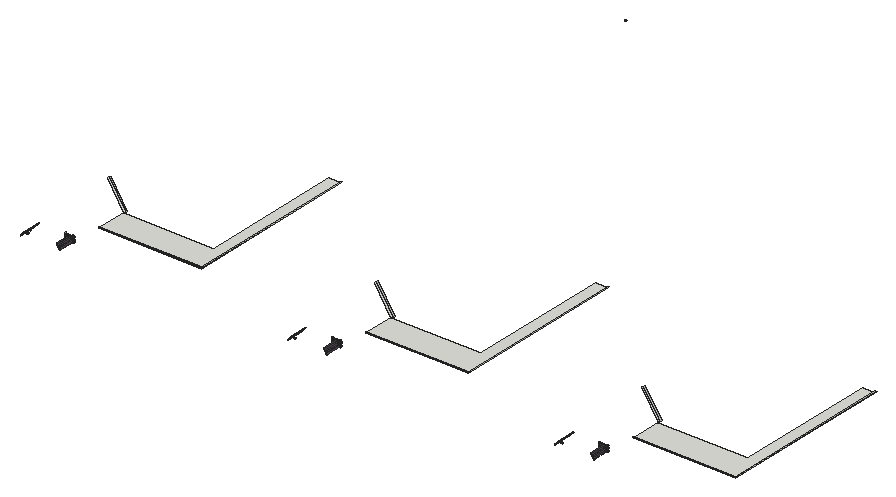
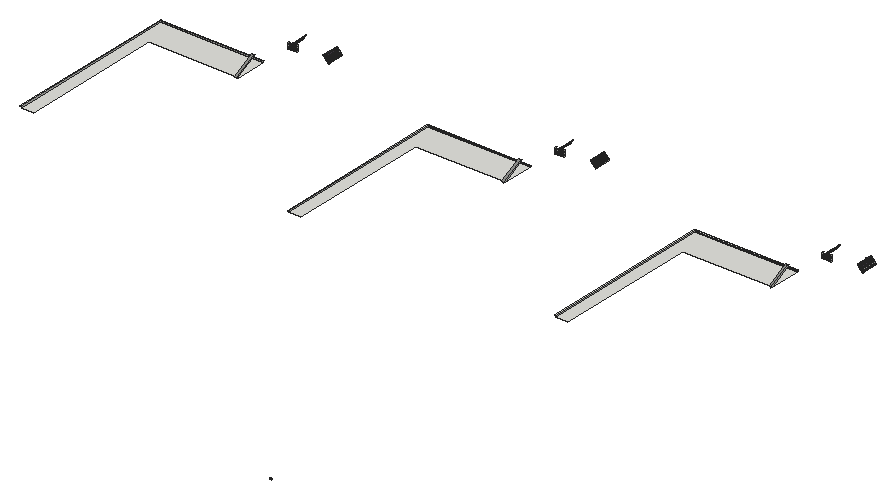
# SketchUp Ruby script. Lengths in inches.
U = 1.inch
M = Sketchup.active_model
def pt(a) = Geom::Point3d.new(a.map { |v| v * U })
def face(e, loops, mat)
  f = e.add_face(loops[0].map { |a| pt(a) })
  loops[1..].each { |l| e.add_face(l.map { |a| pt(a) }).erase! }
  f.material = f.back_material = mat if mat
  f
end
# faces: each face lists its corners as indices into pts; further lists are holes
def faces(e, pts, list, mat = nil) = list.each { |f| face(e, (f[0].is_a?(Array) ? f : [f]).map { |l| l.map { |i| pts[i] } }, mat) }
# xy, xz, yz: faces in a plane at the given z, y or x. An outline is a flat list of corners, or four numbers for a rectangle; further outlines are holes
def ring(l) = l.size == 4 ? [[l[0], l[1]], [l[2], l[1]], [l[2], l[3]], [l[0], l[3]]] : l.each_slice(2).to_a
def flat(e, list, mat, &to3) = list.each { |f| face(e, (f[0].is_a?(Array) ? f : [f]).map { |l| ring(l).map { |u, v| to3.(u, v) } }, mat) }
def xy(e, z, list, mat = nil) = flat(e, list, mat) { |x, y| [x, y, z] }
def xz(e, y, list, mat = nil) = flat(e, list, mat) { |x, z| [x, y, z] }
def yz(e, x, list, mat = nil) = flat(e, list, mat) { |y, z| [x, y, z] }
def lines(e, pts, list) = list.each { |a, b| e.add_line(pt(pts[a]), pt(pts[b])) }
# prism: a flat outline (further loops are holes) pulled along v
def prism(e, loops, v, mat = nil)
  f = face(e, loops, mat); d = Geom::Vector3d.new(v.map { |x| x * U })
  f.pushpull(f.normal.samedirection?(d) ? d.length : -d.length)
end
def box(e, o, s, mat = nil) = prism(e, [[o, [o[0] + s[0], o[1], o[2]], [o[0] + s[0], o[1] + s[1], o[2]], [o[0], o[1] + s[1], o[2]]]], [0, 0, s[2]], mat)
def at(x, y, z, deg = 0) = Geom::Transformation.translation(pt([x, y, z])) * Geom::Transformation.rotation(ORIGIN, Z_AXIS, deg.degrees)
def axes(o, x, y, z) = Geom::Transformation.new([*x, 0, *y, 0, *z, 0, *pt(o).to_a, 1])
def part(name) = M.definitions.add(name)
# library, detail: a bought-in or finely detailed component or shape, given as its bounding box
def library(name, o, s) = part(name).tap { |d| box(d.entities, o, s) }
def detail(e, o, s) = box(e.add_group.entities, o, s)
def put(e, d, t, mat = nil) = e.add_instance(d, t).tap { |i| i.material = mat if mat }
def group(e, t, mat = nil) = e.add_group.tap { |g| g.transformation = t; g.material = mat if mat }.entities
root = M.entities
M.materials.add("[Color M06]").color = [79, 71, 84]
xy(root,366.25,[[578.05,524.25,607.53,526.125],[1464.52,524.25,1494,526.125],[2350.98,524.25,2380.46,526.125]])
xy(root,367.1875,[[611.36,623.84,952.01,623.84,952.01,1201.875,910.57,1201.875,910.57,726.125,611.36,726.125],[1497.82,623.84,1838.47,623.84,1838.47,1201.875,1797.03,1201.875,1797.03,726.125,1497.82,726.125],[2384.28,623.84,2724.93,623.84,2724.93,1201.875,2683.5,1201.875,2683.5,726.125,2384.28,726.125]])
xy(root,369.37,[[578.05,524.25,605.53,526.125],[1464.52,524.25,1491.99,526.125],[2350.98,524.25,2378.45,526.125]])
xy(root,370.27,[[488.53,480.77,490.84,482.33],[1374.99,480.77,1377.3,482.33],[2261.45,480.77,2263.77,482.33]])
xy(root,370.5,[[578.05,524.25,604.81,526.125],[1464.52,524.25,1491.27,526.125],[2350.98,524.25,2377.73,526.125]])
xy(root,370.8125,[[611.36,620.41,952.01,623.84],[952.01,620.41,955.44,623.84],[1497.82,620.41,1838.47,623.84],[1838.47,620.41,1841.91,623.84],[2384.28,620.41,2724.93,623.84],
  [2724.93,620.41,2728.37,623.84],[952.01,623.84,955.44,1201.875],[1838.47,623.84,1841.91,1201.875],[2724.93,623.84,2728.37,1201.875]])
xy(root,372.59,[[488.53,480.77,490.84,482.33],[1374.99,480.77,1377.3,482.33],[2261.45,480.77,2263.77,482.33]])
xy(root,373.62,[[578.05,524.25,602.8,526.125],[1464.52,524.25,1489.27,526.125],[2350.98,524.25,2375.73,526.125]])
xy(root,374.75,[[578.05,524.25,602.08,526.125],[1464.52,524.25,1488.55,526.125],[2350.98,524.25,2375.01,526.125]])
xy(root,377.87,[[578.05,524.25,600.08,526.125],[1464.52,524.25,1486.54,526.125],[2350.98,524.25,2373.01,526.125]])
xy(root,379,[[578.05,524.25,599.36,526.125],[1464.52,524.25,1485.82,526.125],[2350.98,524.25,2372.29,526.125]])
xy(root,382.12,[[578.05,524.25,597.35,526.125],[1464.52,524.25,1483.82,526.125],[2350.98,524.25,2370.28,526.125]])
xy(root,383.25,[[578.05,524.25,596.63,526.125],[1464.52,524.25,1483.1,526.125],[2350.98,524.25,2369.5625,526.125]])
xy(root,384.09,[[494.35,480.14,496.66,480.77],[497.26,480.14,499.58,480.77]])
xz(root,480.77,[[485.59,370.27,485.61,372.59],[485.61,370.27,487.9,372.59],[1372.05,370.27,1372.08,372.59],[1372.08,370.27,1374.37,372.59],[2258.52,370.27,2258.54,372.59],
  [2258.54,370.27,2260.83,372.59]])
xz(root,482.33,[[488.53,370.27,490.84,372.59],[1374.99,370.27,1377.3,372.59],[2261.45,370.27,2263.77,372.59]])
xz(root,519.6875,[[605.875,368.02,605.82,368.11,606.1875,368.34,606.24,368.25],[1492.34,368.02,1492.28,368.11,1492.65,368.34,1492.71,368.25],[2378.8,368.02,2378.75,368.11,2379.11,368.34,2379.17,368.25],[603.55,371.65,603.49,371.74,603.86,371.97,603.92,371.88],[1490.01,371.65,1489.96,371.74,1490.32,371.97,1490.38,371.88],
  [2376.48,371.65,2376.42,371.74,2376.79,371.97,2376.84,371.88],[601.36,375.07,601.3,375.16,601.67,375.39,601.72,375.3],[1487.82,375.07,1487.76,375.16,1488.13,375.39,1488.1875,375.3],[2374.28,375.07,2374.23,375.16,2374.59,375.39,2374.65,375.3],[599.16,378.49,599.11,378.58,599.47,378.8125,599.53,378.72],
  [1485.625,378.49,1485.57,378.58,1485.9375,378.8125,1485.99,378.72],[2372.09,378.49,2372.03,378.58,2372.4,378.8125,2372.46,378.72],[596.97,381.91,596.91,382,597.28,382.23,597.34,382.14],[1483.43,381.91,1483.38,382,1483.75,382.23,1483.8,382.14],[2369.9,381.91,2369.84,382,2370.21,382.23,2370.27,382.14]])
xz(root,521.5625,[[475.14,366.22,477.57,368.8,477.11,369.23,474.6875,366.65],[1361.61,366.22,1364.03,368.8,1363.57,369.23,1361.15,366.65],[2248.07,366.22,2250.49,368.8,2250.04,369.23,2247.62,366.65],[605.1875,369.09,603.55,371.65,603.92,371.88,605.55,369.33],[1491.65,369.09,1490.01,371.65,1490.38,371.88,1492.02,369.33],
  [2378.11,369.09,2376.48,371.65,2376.84,371.88,2378.48,369.33],[478.44,369.73,480.86,372.3,480.41,372.73,477.99,370.16],[1364.91,369.73,1367.33,372.3,1366.87,372.73,1364.45,370.16],[2251.37,369.73,2253.79,372.3,2253.34,372.73,2250.92,370.16],[602.99,372.51,601.36,375.07,601.72,375.3,603.36,372.75],
  [1489.46,372.51,1487.82,375.07,1488.1875,375.3,1489.83,372.75],[2375.92,372.51,2374.28,375.07,2374.65,375.3,2376.29,372.75],[481.74,373.23,484.16,375.81,483.71,376.23,481.29,373.66],[1368.21,373.23,1370.625,375.81,1370.17,376.23,1367.75,373.66],[2254.67,373.23,2257.09,375.81,2256.64,376.23,2254.21,373.66],
  [600.8,375.93,599.16,378.49,599.53,378.72,601.17,376.17],[1487.26,375.93,1485.625,378.49,1485.99,378.72,1487.63,376.17],[2373.73,375.93,2372.09,378.49,2372.46,378.72,2374.1,376.17],[485.04,376.74,487.46,379.31,487.01,379.74,484.58,377.17],[1371.5,376.74,1373.92,379.31,1373.47,379.74,1371.05,377.17],
  [2257.97,376.74,2260.39,379.31,2259.93,379.74,2257.51,377.17],[598.61,379.35,596.97,381.91,597.34,382.14,598.98,379.59],[1485.07,379.35,1483.43,381.91,1483.8,382.14,1485.44,379.59],[2371.54,379.35,2369.9,381.91,2370.27,382.14,2371.9,379.59],[488.34,380.24,490.76,382.8125,490.3,383.24,487.88,380.67],
  [1374.8,380.24,1377.22,382.8125,1376.77,383.24,1374.35,380.67],[2261.27,380.24,2263.6875,382.8125,2263.23,383.24,2260.8125,380.67],[596.42,382.77,594.78,385.33,595.15,385.56,596.78,383.01],[1482.88,382.77,1481.24,385.33,1481.61,385.56,1483.25,383.01],[2369.34,382.77,2367.71,385.33,2368.07,385.56,2369.71,383.01],
  [491.64,383.75,494.06,386.32,493.6,386.75,491.18,384.17],[1378.1,383.75,1380.52,386.32,1380.07,386.75,1377.65,384.17],[2264.56,383.75,2266.99,386.32,2266.53,386.75,2264.11,384.17]])
xz(root,524.25,[[578.05,366.25,607.53,366.25,605.53,369.37,578.05,369.37],[1464.52,366.25,1494,366.25,1491.99,369.37,1464.52,369.37],[2350.98,366.25,2380.46,366.25,2378.45,369.37,2350.98,369.37],[578.05,370.5,604.81,370.5,602.8,373.62,578.05,373.62],[1464.52,370.5,1491.27,370.5,1489.27,373.62,1464.52,373.62],
  [2350.98,370.5,2377.73,370.5,2375.73,373.62,2350.98,373.62],[578.05,374.75,602.08,374.75,600.08,377.87,578.05,377.87],[1464.52,374.75,1488.55,374.75,1486.54,377.87,1464.52,377.87],[2350.98,374.75,2375.01,374.75,2373.01,377.87,2350.98,377.87],[578.05,379,599.36,379,597.35,382.12,578.05,382.12],
  [1464.52,379,1485.82,379,1483.82,382.12,1464.52,382.12],[2350.98,379,2372.29,379,2370.28,382.12,2350.98,382.12],[578.05,383.25,596.63,383.25,594.63,386.37,578.05,386.37],[1464.52,383.25,1483.1,383.25,1481.09,386.37,1464.52,386.37],[2350.98,383.25,2369.5625,383.25,2367.56,386.37,2350.98,386.37]],"[Color M06]")
xz(root,526.125,[[609.02,368.17,609.02,369.37,608.25,369.37],[1495.49,368.17,1495.49,369.37,1494.72,369.37],[2381.95,368.17,2381.95,369.37,2381.18,369.37],[578.05,369.37,605.53,369.37,604.81,370.5,578.05,370.5],[1464.52,369.37,1491.99,369.37,1491.27,370.5,1464.52,370.5],
  [2350.98,369.37,2378.45,369.37,2377.73,370.5,2350.98,370.5],[604.81,370.5,607.53,370.5,605.53,373.62,602.8,373.62],[1491.27,370.5,1494,370.5,1491.99,373.62,1489.27,373.62],[2377.73,370.5,2380.46,370.5,2378.45,373.62,2375.73,373.62],[578.05,373.62,602.8,373.62,602.08,374.75,578.05,374.75],
  [1464.52,373.62,1489.27,373.62,1488.55,374.75,1464.52,374.75],[2350.98,373.62,2375.73,373.62,2375.01,374.75,2350.98,374.75],[604.81,374.75,607.53,374.75,605.53,377.87,602.8,377.87],[1491.27,374.75,1494,374.75,1491.99,377.87,1489.27,377.87],[2377.73,374.75,2380.46,374.75,2378.45,377.87,2375.73,377.87],
  [578.05,377.87,600.08,377.87,599.36,379,578.05,379],[1464.52,377.87,1486.54,377.87,1485.82,379,1464.52,379],[2350.98,377.87,2373.01,377.87,2372.29,379,2350.98,379],[604.81,379,607.53,379,605.53,382.12,602.8,382.12],[1491.27,379,1494,379,1491.99,382.12,1489.27,382.12],
  [2377.73,379,2380.46,379,2378.45,382.12,2375.73,382.12],[578.05,382.12,597.35,382.12,596.63,383.25,578.05,383.25],[1464.52,382.12,1483.82,382.12,1483.1,383.25,1464.52,383.25],[2350.98,382.12,2370.28,382.12,2369.5625,383.25,2350.98,383.25],[604.81,383.25,607.53,383.25,605.53,386.37,602.8,386.37],
  [1491.27,383.25,1494,383.25,1491.99,386.37,1489.27,386.37],[2377.73,383.25,2380.46,383.25,2378.45,386.37,2375.73,386.37]])
xz(root,623.84,[[611.36,367.1875,952.01,370.8125],[1497.82,367.1875,1838.47,370.8125],[2384.28,367.1875,2724.93,370.8125]])
xz(root,726.125,[[611.36,366.85,611.36,367.1875,611.88,367.1875],[1497.82,366.85,1497.82,367.1875,1498.34,367.1875],[2384.28,366.85,2384.28,367.1875,2384.81,367.1875],[611.88,367.1875,612.42,367.53,612.64,367.1875],[1498.34,367.1875,1498.89,367.53,1499.11,367.1875],
  [2384.81,367.1875,2385.35,367.53,2385.57,367.1875]])
xz(root,732.2,[[612.42,367.53,557.61,453.03,562.87,456.41,617.68,370.91],[1498.89,367.53,1444.07,453.03,1449.33,456.41,1504.15,370.91],[2385.35,367.53,2330.53,453.03,2335.8,456.41,2390.61,370.91]])
xz(root,2332.13,[[989.79,366.33,990.38,366.96,989.79,366.96],[988.21,367.46,988.26,367.46,989.1875,368.45,989.1875,368.5],[988.26,367.46,989.1875,367.46,989.1875,368.45],[989.79,367.46,989.84,367.46,992,369.77,990.4375,369.77,989.79,369.08],[989.84,367.46,990.85,367.46,992.1,368.78,992.1,369.77,992,369.77],
  [990.85,367.46,992.1,367.46,992.1,368.78],[992.7,367.7,994.64,369.77,993.03,369.77,992.7,369.42],[995.61,368,997.27,369.77,995.61,369.77]])
xz(root,2332.13,[[992.7,367.46,995.01,367.46,995.01,369.77,994.64,369.77,992.7,367.7]],"[Color M06]")
yz(root,488.53,[[480.77,370.27,482.33,372.59]])
yz(root,490.84,[[480.77,370.27,482.33,372.59]])
yz(root,499.58,[[480.14,384.09,480.77,386.4]])
yz(root,578.05,[[524.25,366.25,526.125,369.37],[524.25,370.5,526.125,373.62],[524.25,374.75,526.125,377.87],[524.25,379,526.125,382.12],[524.25,383.25,526.125,386.37]])
yz(root,952.01,[[623.84,367.1875,1201.875,370.8125]])
yz(root,1374.99,[[480.77,370.27,482.33,372.59]])
yz(root,1377.3,[[480.77,370.27,482.33,372.59]])
yz(root,1464.52,[[524.25,366.25,526.125,369.37],[524.25,370.5,526.125,373.62],[524.25,374.75,526.125,377.87],[524.25,379,526.125,382.12],[524.25,383.25,526.125,386.37]])
yz(root,1838.47,[[623.84,367.1875,1201.875,370.8125]])
yz(root,2261.45,[[480.77,370.27,482.33,372.59]])
yz(root,2263.77,[[480.77,370.27,482.33,372.59]])
yz(root,2350.98,[[524.25,366.25,526.125,369.37],[524.25,370.5,526.125,373.62],[524.25,374.75,526.125,377.87],[524.25,379,526.125,382.12],[524.25,383.25,526.125,386.37]])
yz(root,2724.93,[[623.84,367.1875,1201.875,370.8125]])
p = [[474.6875,467.1875,366.65],[474.6875,521.5625,366.65],[475.14,521.5625,366.22],[475.14,467.1875,366.22],[477.57,521.5625,368.8],[477.57,467.1875,368.8],
  [1361.15,467.1875,366.65],[1361.15,521.5625,366.65],[1361.61,521.5625,366.22],[1361.61,467.1875,366.22],[1364.03,521.5625,368.8],[1364.03,467.1875,368.8],
  [2247.62,467.1875,366.65],[2247.62,521.5625,366.65],[2248.07,521.5625,366.22],[2248.07,467.1875,366.22],[2250.49,521.5625,368.8],[2250.49,467.1875,368.8],
  [612.42,726.125,367.53],[557.61,726.125,453.03],[557.61,732.2,453.03],[612.42,732.2,367.53],[1498.89,726.125,367.53],[1444.07,726.125,453.03],
  [1444.07,732.2,453.03],[1498.89,732.2,367.53],[2385.35,726.125,367.53],[2330.53,726.125,453.03],[2330.53,732.2,453.03],[2385.35,732.2,367.53],
  [606.24,519.6875,368.25],[606.24,521.5625,368.25],[605.875,521.5625,368.02],[605.875,519.6875,368.02],[1492.71,519.6875,368.25],[1492.71,521.5625,368.25],
  [1492.34,521.5625,368.02],[1492.34,519.6875,368.02],[2379.17,519.6875,368.25],[2379.17,521.5625,368.25],[2378.8,521.5625,368.02],[2378.8,519.6875,368.02],
  [606.1875,467.1875,368.34],[606.1875,519.6875,368.34],[605.82,519.6875,368.11],[605.82,467.1875,368.11],[1492.65,467.1875,368.34],[1492.65,519.6875,368.34],
  [1492.28,519.6875,368.11],[1492.28,467.1875,368.11],[2379.11,467.1875,368.34],[2379.11,519.6875,368.34],[2378.75,519.6875,368.11],[2378.75,467.1875,368.11],
  [477.11,521.5625,369.23],[477.11,467.1875,369.23],[1363.57,521.5625,369.23],[1363.57,467.1875,369.23],[2250.04,521.5625,369.23],[2250.04,467.1875,369.23],
  [603.49,467.1875,371.74],[603.49,519.6875,371.74],[603.55,519.6875,371.65],[603.55,521.5625,371.65],[605.1875,521.5625,369.09],[605.1875,467.1875,369.09],
  [605.55,521.5625,369.33],[605.55,467.1875,369.33],[1489.96,467.1875,371.74],[1489.96,519.6875,371.74],[1490.01,519.6875,371.65],[1490.01,521.5625,371.65],
  [1491.65,521.5625,369.09],[1491.65,467.1875,369.09],[1492.02,521.5625,369.33],[1492.02,467.1875,369.33],[2376.42,467.1875,371.74],[2376.42,519.6875,371.74],
  [2376.48,519.6875,371.65],[2376.48,521.5625,371.65],[2378.11,521.5625,369.09],[2378.11,467.1875,369.09],[2378.48,521.5625,369.33],[2378.48,467.1875,369.33],
  [477.99,521.5625,370.16],[477.99,467.1875,370.16],[1364.45,521.5625,370.16],[1364.45,467.1875,370.16],[2250.92,521.5625,370.16],[2250.92,467.1875,370.16],
  [478.44,521.5625,369.73],[478.44,467.1875,369.73],[480.86,521.5625,372.3],[480.86,467.1875,372.3],[1364.91,521.5625,369.73],[1364.91,467.1875,369.73],
  [1367.33,521.5625,372.3],[1367.33,467.1875,372.3],[2251.37,521.5625,369.73],[2251.37,467.1875,369.73],[2253.79,521.5625,372.3],[2253.79,467.1875,372.3],
  [602.8,526.125,373.62],[604.81,526.125,370.5],[604.81,524.25,370.5],[602.8,524.25,373.62],[1489.27,526.125,373.62],[1491.27,526.125,370.5],
  [1491.27,524.25,370.5],[1489.27,524.25,373.62],[2375.73,526.125,373.62],[2377.73,526.125,370.5],[2377.73,524.25,370.5],[2375.73,524.25,373.62],
  [603.92,519.6875,371.88],[603.92,521.5625,371.88],[1490.38,519.6875,371.88],[1490.38,521.5625,371.88],[2376.84,519.6875,371.88],[2376.84,521.5625,371.88],
  [603.86,467.1875,371.97],[603.86,519.6875,371.97],[1490.32,467.1875,371.97],[1490.32,519.6875,371.97],[2376.79,467.1875,371.97],[2376.79,519.6875,371.97],
  [480.41,521.5625,372.73],[480.41,467.1875,372.73],[1366.87,521.5625,372.73],[1366.87,467.1875,372.73],[2253.34,521.5625,372.73],[2253.34,467.1875,372.73],
  [601.3,467.1875,375.16],[601.3,519.6875,375.16],[601.36,519.6875,375.07],[601.36,521.5625,375.07],[602.99,521.5625,372.51],[602.99,467.1875,372.51],
  [603.36,521.5625,372.75],[603.36,467.1875,372.75],[1487.76,467.1875,375.16],[1487.76,519.6875,375.16],[1487.82,519.6875,375.07],[1487.82,521.5625,375.07],
  [1489.46,521.5625,372.51],[1489.46,467.1875,372.51],[1489.83,521.5625,372.75],[1489.83,467.1875,372.75],[2374.23,467.1875,375.16],[2374.23,519.6875,375.16],
  [2374.28,519.6875,375.07],[2374.28,521.5625,375.07],[2375.92,521.5625,372.51],[2375.92,467.1875,372.51],[2376.29,521.5625,372.75],[2376.29,467.1875,372.75],
  [481.29,521.5625,373.66],[481.29,467.1875,373.66],[1367.75,521.5625,373.66],[1367.75,467.1875,373.66],[2254.21,521.5625,373.66],[2254.21,467.1875,373.66],
  [481.74,521.5625,373.23],[481.74,467.1875,373.23],[484.16,521.5625,375.81],[484.16,467.1875,375.81],[1368.21,521.5625,373.23],[1368.21,467.1875,373.23],
  [1370.625,521.5625,375.81],[1370.625,467.1875,375.81],[2254.67,521.5625,373.23],[2254.67,467.1875,373.23],[2257.09,521.5625,375.81],[2257.09,467.1875,375.81],
  [601.72,519.6875,375.3],[601.72,521.5625,375.3],[1488.1875,519.6875,375.3],[1488.1875,521.5625,375.3],[2374.65,519.6875,375.3],[2374.65,521.5625,375.3],
  [601.67,467.1875,375.39],[601.67,519.6875,375.39],[1488.13,467.1875,375.39],[1488.13,519.6875,375.39],[2374.59,467.1875,375.39],[2374.59,519.6875,375.39],
  [483.71,521.5625,376.23],[483.71,467.1875,376.23],[1370.17,521.5625,376.23],[1370.17,467.1875,376.23],[2256.64,521.5625,376.23],[2256.64,467.1875,376.23],
  [599.11,467.1875,378.58],[599.11,519.6875,378.58],[599.16,519.6875,378.49],[599.16,521.5625,378.49],[600.8,521.5625,375.93],[600.8,467.1875,375.93],
  [601.17,521.5625,376.17],[601.17,467.1875,376.17],[1485.57,467.1875,378.58],[1485.57,519.6875,378.58],[1485.625,519.6875,378.49],[1485.625,521.5625,378.49],
  [1487.26,521.5625,375.93],[1487.26,467.1875,375.93],[1487.63,521.5625,376.17],[1487.63,467.1875,376.17],[2372.03,467.1875,378.58],[2372.03,519.6875,378.58],
  [2372.09,519.6875,378.49],[2372.09,521.5625,378.49],[2373.73,521.5625,375.93],[2373.73,467.1875,375.93],[2374.1,521.5625,376.17],[2374.1,467.1875,376.17],
  [484.58,521.5625,377.17],[484.58,467.1875,377.17],[1371.05,521.5625,377.17],[1371.05,467.1875,377.17],[2257.51,521.5625,377.17],[2257.51,467.1875,377.17],
  [485.04,521.5625,376.74],[485.04,467.1875,376.74],[487.46,521.5625,379.31],[487.46,467.1875,379.31],[1371.5,521.5625,376.74],[1371.5,467.1875,376.74],
  [1373.92,521.5625,379.31],[1373.92,467.1875,379.31],[2257.97,521.5625,376.74],[2257.97,467.1875,376.74],[2260.39,521.5625,379.31],[2260.39,467.1875,379.31],
  [599.53,519.6875,378.72],[599.53,521.5625,378.72],[1485.99,519.6875,378.72],[1485.99,521.5625,378.72],[2372.46,519.6875,378.72],[2372.46,521.5625,378.72],
  [599.47,467.1875,378.8125],[599.47,519.6875,378.8125],[1485.9375,467.1875,378.8125],[1485.9375,519.6875,378.8125],[2372.4,467.1875,378.8125],[2372.4,519.6875,378.8125],
  [487.01,521.5625,379.74],[487.01,467.1875,379.74],[1373.47,521.5625,379.74],[1373.47,467.1875,379.74],[2259.93,521.5625,379.74],[2259.93,467.1875,379.74],
  [596.91,467.1875,382],[596.91,519.6875,382],[596.97,519.6875,381.91],[596.97,521.5625,381.91],[598.61,521.5625,379.35],[598.61,467.1875,379.35],
  [598.98,521.5625,379.59],[598.98,467.1875,379.59],[1483.38,467.1875,382],[1483.38,519.6875,382],[1483.43,519.6875,381.91],[1483.43,521.5625,381.91],
  [1485.07,521.5625,379.35],[1485.07,467.1875,379.35],[1485.44,521.5625,379.59],[1485.44,467.1875,379.59],[2369.84,467.1875,382],[2369.84,519.6875,382],
  [2369.9,519.6875,381.91],[2369.9,521.5625,381.91],[2371.54,521.5625,379.35],[2371.54,467.1875,379.35],[2371.9,521.5625,379.59],[2371.9,467.1875,379.59],
  [487.88,521.5625,380.67],[487.88,467.1875,380.67],[1374.35,521.5625,380.67],[1374.35,467.1875,380.67],[2260.8125,521.5625,380.67],[2260.8125,467.1875,380.67],
  [488.34,521.5625,380.24],[488.34,467.1875,380.24],[490.76,521.5625,382.8125],[490.76,467.1875,382.8125],[1374.8,521.5625,380.24],[1374.8,467.1875,380.24],
  [1377.22,521.5625,382.8125],[1377.22,467.1875,382.8125],[2261.27,521.5625,380.24],[2261.27,467.1875,380.24],[2263.6875,521.5625,382.8125],[2263.6875,467.1875,382.8125],
  [597.34,519.6875,382.14],[597.34,521.5625,382.14],[1483.8,519.6875,382.14],[1483.8,521.5625,382.14],[2370.27,519.6875,382.14],[2370.27,521.5625,382.14],
  [597.28,467.1875,382.23],[597.28,519.6875,382.23],[1483.75,467.1875,382.23],[1483.75,519.6875,382.23],[2370.21,467.1875,382.23],[2370.21,519.6875,382.23],
  [490.3,521.5625,383.24],[490.3,467.1875,383.24],[594.72,467.1875,385.42],[594.72,519.6875,385.42],[594.78,519.6875,385.33],[594.78,521.5625,385.33],
  [596.42,521.5625,382.77],[596.42,467.1875,382.77],[596.78,521.5625,383.01],[596.78,467.1875,383.01],[1376.77,521.5625,383.24],[1376.77,467.1875,383.24],
  [1481.18,467.1875,385.42],[1481.18,519.6875,385.42],[1481.24,519.6875,385.33],[1481.24,521.5625,385.33],[1482.88,521.5625,382.77],[1482.88,467.1875,382.77],
  [1483.25,521.5625,383.01],[1483.25,467.1875,383.01],[2263.23,521.5625,383.24],[2263.23,467.1875,383.24],[2367.65,467.1875,385.42],[2367.65,519.6875,385.42],
  [2367.71,519.6875,385.33],[2367.71,521.5625,385.33],[2369.34,521.5625,382.77],[2369.34,467.1875,382.77],[2369.71,521.5625,383.01],[2369.71,467.1875,383.01],
  [491.18,521.5625,384.17],[491.18,467.1875,384.17],[1377.65,521.5625,384.17],[1377.65,467.1875,384.17],[2264.11,521.5625,384.17],[2264.11,467.1875,384.17],
  [491.64,521.5625,383.75],[491.64,480.14,383.75],[491.64,467.1875,383.75],[494.06,521.5625,386.32],[494.06,467.1875,386.32],[1378.1,521.5625,383.75],
  [1378.1,480.14,383.75],[1378.1,467.1875,383.75],[1380.52,521.5625,386.32],[1380.52,467.1875,386.32],[2264.56,521.5625,383.75],[2264.57,480.14,383.75],
  [2264.56,467.1875,383.75],[2266.99,521.5625,386.32],[2266.99,467.1875,386.32],[1495.49,526.125,366.25],[1494,526.125,366.25],[1495.49,526.125,368.17],
  [1491.99,526.125,369.37],[1494.72,526.125,369.37],[1491.27,526.125,374.75],[1488.55,526.125,374.75],[1486.54,526.125,377.87],[1489.27,526.125,377.87],
  [1486.54,526.125,382.12],[1489.27,526.125,382.12],[1488.55,526.125,379],[1485.82,526.125,379],[1491.27,526.125,379],[1483.82,526.125,382.12],
  [1488.55,526.125,383.25],[1485.82,526.125,383.25],[1491.27,526.125,383.25],[1483.1,526.125,383.25],[2381.95,526.125,368.17],[2381.95,526.125,366.25],
  [2380.46,526.125,366.25],[2378.45,526.125,369.37],[2381.18,526.125,369.37],[2372.29,526.125,383.25],[2369.5625,526.125,383.25],[2377.73,526.125,383.25],
  [2375.01,526.125,383.25],[2373.01,526.125,377.87],[2375.73,526.125,377.87],[2377.73,526.125,374.75],[2375.01,526.125,374.75],[2375.01,526.125,379],
  [2372.29,526.125,379],[2377.73,526.125,379],[2373.01,526.125,382.12],[2375.73,526.125,382.12],[2370.28,526.125,382.12],[597.35,526.125,382.12],
  [600.08,526.125,382.12],[604.81,526.125,379],[602.08,526.125,379],[602.8,526.125,382.12],[599.36,526.125,379],[600.08,526.125,377.87],
  [602.8,526.125,377.87],[604.81,526.125,374.75],[602.08,526.125,374.75],[609.02,526.125,368.17],[609.02,526.125,366.25],[605.53,526.125,369.37],
  [608.25,526.125,369.37],[607.53,526.125,366.25],[602.08,526.125,383.25],[599.36,526.125,383.25],[596.63,526.125,383.25],[604.81,526.125,383.25],
  [987.2,2332.13,370.27],[986.875,2332.13,370.27],[992.1,2332.13,372.59],[992.1,2332.13,371.6],[989.79,2332.13,369.08],[989.79,2332.13,369.14],
  [994.64,2332.13,375.4],[992.7,2332.13,373.33],[995.61,2332.13,375.4],[995.68,2332.13,375.4],[992.7,2332.13,372.23],[992.7,2332.13,372.59],
  [993.03,2332.13,372.59],[989.79,2332.13,369.77],[990.38,2332.13,369.77],[990.85,2332.13,370.27],[989.79,2332.13,370.27],[990.4375,2332.13,369.77],
  [992,2332.13,372.59],[987.74,2332.13,366.96],[987.79,2332.13,366.96],[986.875,2332.13,366.05],[986.875,2332.13,366.96],[995.01,2332.13,375.4],
  [995.01,2332.13,374.69],[993.55,2332.13,373.09],[993.5,2332.13,373.09],[997.92,2332.13,378.15],[997.92,2332.13,377.73],[1002.55,2332.13,383.65],
  [1001.43,2332.13,382.46],[1004.35,2332.13,384.55],[1004.35,2332.13,385.57],[997.92,2332.13,378.59],[997.74,2332.13,378.59],[995.61,2332.13,375.84],
  [995.61,2332.13,376.375],[997.27,2332.13,378.15],[998.73,2332.13,378.59],[998.52,2332.13,378.59],[1000.83,2332.13,381.34],[1000.38,2332.13,381.34],
  [1003.5,2332.13,383.65],[996.14,2332.13,375.84],[1000.83,2332.13,381.82],[996.15,2332.13,378.59],[996.14,2332.13,378.59],[998.52,2332.13,380.9],
  [1000.83,2332.13,380.9],[1000.83,2332.13,380.82],[997.92,2332.13,378.78],[1003.75,2332.13,384.93],[1003.75,2332.13,384.09],[998.74,2332.13,381.34],
  [998.73,2332.13,381.34],[1002.96,2332.13,384.09],[1001.43,2332.13,381.46],[992.7,2332.13,373.09],[986.875,2332.13,365.99],[995.61,2332.13,375.33],
  [995.01,2332.13,374.63]]
faces(root,p,[[0,1,2,3],[6,7,8,9],[12,13,14,15],[18,19,20,21],[22,23,24,25],[26,27,28,29],[30,31,32,33],[34,35,36,37],
  [38,39,40,41],[42,43,44,45],[46,47,48,49],[50,51,52,53],[54,55,5,4],[56,57,11,10],[58,59,17,16],[66,67,65,64],
  [74,75,73,72],[82,83,81,80],[85,84,90,91],[87,86,94,95],[89,88,98,99],[102,103,104,105],[106,107,108,109],[110,111,112,113],
  [114,115,63,62],[116,117,71,70],[118,119,79,78],[120,121,61,60],[122,123,69,68],[124,125,77,76],[126,127,93,92],[128,129,97,96],
  [130,131,101,100],[138,139,137,136],[146,147,145,144],[154,155,153,152],[157,156,162,163],[159,158,166,167],[161,160,170,171],[174,175,135,134],
  [176,177,143,142],[178,179,151,150],[180,181,133,132],[182,183,141,140],[184,185,149,148],[186,187,165,164],[188,189,169,168],[190,191,173,172],
  [198,199,197,196],[206,207,205,204],[214,215,213,212],[217,216,222,223],[219,218,226,227],[221,220,230,231],[234,235,195,194],[236,237,203,202],
  [238,239,211,210],[240,241,193,192],[242,243,201,200],[244,245,209,208],[258,259,257,256],[266,267,265,264],[274,275,273,272],[277,276,282,283],
  [279,278,286,287],[281,280,290,291],[294,295,255,254],[296,297,263,262],[298,299,271,270],[300,301,253,252],[302,303,261,260],[304,305,269,268],
  [306,307,285,284],[314,315,313,312],[316,317,289,288],[324,325,323,322],[326,327,293,292],[334,335,333,332],[337,336,342,343,344],[339,338,347,348,349],
  [341,340,352,353,354]])
faces(root,p,[[2,4,5,3],[8,10,11,9],[14,16,17,15],[60,61,62,63,64,65],[68,69,70,71,72,73],[76,77,78,79,80,81],[54,84,85,55],[56,86,87,57],
  [58,88,89,59],[90,92,93,91],[94,96,97,95],[98,100,101,99],[132,133,134,135,136,137],[140,141,142,143,144,145],[148,149,150,151,152,153],[126,156,157,127],
  [128,158,159,129],[130,160,161,131],[162,164,165,163],[166,168,169,167],[170,172,173,171],[192,193,194,195,196,197],[200,201,202,203,204,205],[208,209,210,211,212,213],
  [186,216,217,187],[188,218,219,189],[190,220,221,191],[222,224,225,223],[226,228,229,227],[230,232,233,231],[246,247,225,224],[248,249,229,228],
  [250,251,233,232],[252,253,254,255,256,257],[260,261,262,263,264,265],[268,269,270,271,272,273],[246,276,277,247],[248,278,279,249],[250,280,281,251],[282,284,285,283],
  [286,288,289,287],[290,292,293,291],[308,309,310,311,312,313],[318,319,320,321,322,323],[328,329,330,331,332,333],[306,336,337,307],[316,338,339,317],[326,340,341,327],
  [342,345,346,344,343],[347,350,351,349,348],[352,355,356,354,353]],"[Color M06]")
lines(root,p,[[357,358],[359,357],[360,361],[362,363],[364,365],[366,367],[368,369],[370,368],[371,366],[372,373],[374,372],[373,375],
  [376,377],[377,378],[379,380],[381,382],[383,384],[384,381],[385,386],[387,388],[389,390],[391,389],[392,393],[394,392],
  [395,396],[397,398],[396,399],[398,400],[401,402],[403,404],[405,406],[407,408],[406,409],[410,411],[411,412],[413,410],
  [414,415],[416,417],[418,419],[420,421],[422,423],[424,425],[425,426],[427,428],[419,427],[429,430],[428,431],[432,416],
  [433,434],[435,436],[436,433],[437,438],[439,440],[441,442],[443,444],[445,446],[447,448],[449,450],[451,450],[452,453],
  [451,441],[454,455],[443,456],[457,449],[458,454],[459,460],[461,462],[462,463],[464,447],[465,466],[467,468],[466,469],
  [455,467],[470,444],[471,421],[420,437],[472,435],[473,422],[440,471],[438,474]])
